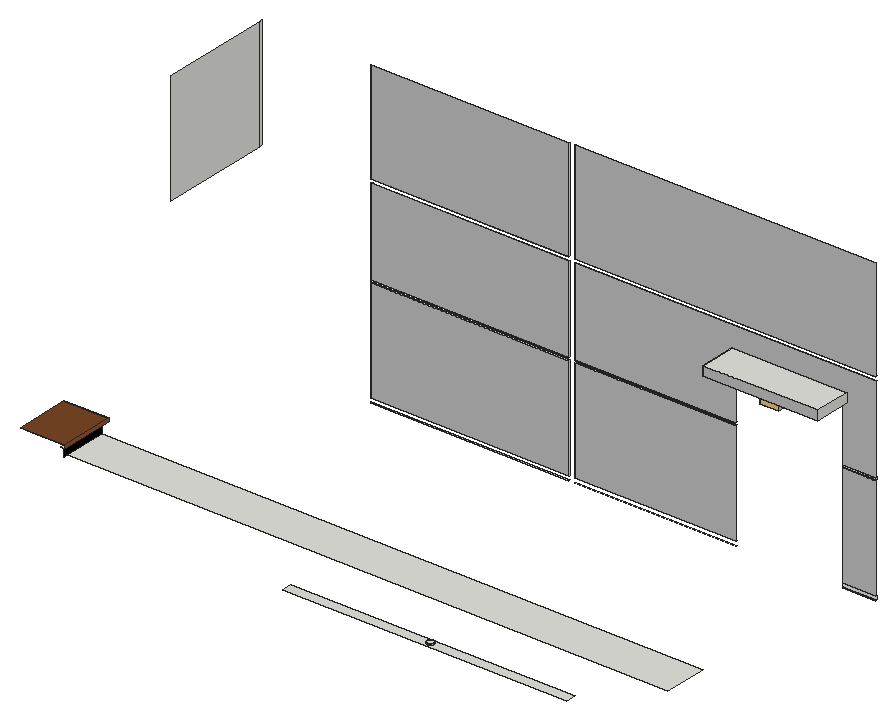
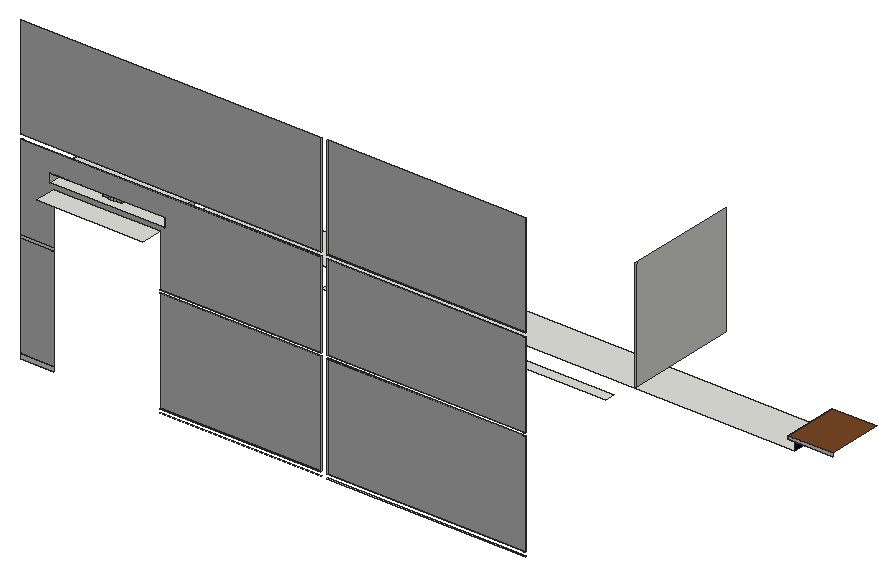
# SketchUp Ruby script. Lengths in inches.
U = 1.inch
M = Sketchup.active_model
def pt(a) = Geom::Point3d.new(a.map { |v| v * U })
def face(e, loops, mat)
  f = e.add_face(loops[0].map { |a| pt(a) })
  loops[1..].each { |l| e.add_face(l.map { |a| pt(a) }).erase! }
  f.material = f.back_material = mat if mat
  f
end
# faces: each face lists its corners as indices into pts; further lists are holes
def faces(e, pts, list, mat = nil) = list.each { |f| face(e, (f[0].is_a?(Array) ? f : [f]).map { |l| l.map { |i| pts[i] } }, mat) }
# xy, xz, yz: faces in a plane at the given z, y or x. An outline is a flat list of corners, or four numbers for a rectangle; further outlines are holes
def ring(l) = l.size == 4 ? [[l[0], l[1]], [l[2], l[1]], [l[2], l[3]], [l[0], l[3]]] : l.each_slice(2).to_a
def flat(e, list, mat, &to3) = list.each { |f| face(e, (f[0].is_a?(Array) ? f : [f]).map { |l| ring(l).map { |u, v| to3.(u, v) } }, mat) }
def xy(e, z, list, mat = nil) = flat(e, list, mat) { |x, y| [x, y, z] }
def xz(e, y, list, mat = nil) = flat(e, list, mat) { |x, z| [x, y, z] }
def yz(e, x, list, mat = nil) = flat(e, list, mat) { |y, z| [x, y, z] }
def lines(e, pts, list) = list.each { |a, b| e.add_line(pt(pts[a]), pt(pts[b])) }
# prism: a flat outline (further loops are holes) pulled along v
def prism(e, loops, v, mat = nil)
  f = face(e, loops, mat); d = Geom::Vector3d.new(v.map { |x| x * U })
  f.pushpull(f.normal.samedirection?(d) ? d.length : -d.length)
end
def box(e, o, s, mat = nil) = prism(e, [[o, [o[0] + s[0], o[1], o[2]], [o[0] + s[0], o[1] + s[1], o[2]], [o[0], o[1] + s[1], o[2]]]], [0, 0, s[2]], mat)
def at(x, y, z, deg = 0) = Geom::Transformation.translation(pt([x, y, z])) * Geom::Transformation.rotation(ORIGIN, Z_AXIS, deg.degrees)
def axes(o, x, y, z) = Geom::Transformation.new([*x, 0, *y, 0, *z, 0, *pt(o).to_a, 1])
def part(name) = M.definitions.add(name)
# library, detail: a bought-in or finely detailed component or shape, given as its bounding box
def library(name, o, s) = part(name).tap { |d| box(d.entities, o, s) }
def detail(e, o, s) = box(e.add_group.entities, o, s)
def put(e, d, t, mat = nil) = e.add_instance(d, t).tap { |i| i.material = mat if mat }
def group(e, t, mat = nil) = e.add_group.tap { |g| g.transformation = t; g.material = mat if mat }.entities
root = M.entities
M.materials.add("[0042_Sienna]1").color = [160, 82, 45]
M.materials.add("[0131_Silver]").color = [192, 192, 192]
M.materials.add("[0137_Black]").color = [0, 0, 0]
M.materials.add("[Wood Veneer 01]").color = [120, 70, 37]
c1 = library("A$C06767DEF\#1",[-8.3,1.21,0],[7.09,7.09,5.51])
xy(root,49.75,[[[765.78,333.31,873.91,337.06],[820.37,334.03,820.71,334.07,821.03,334.2,821.3,334.41,821.51,334.68,821.64,335,821.68,335.34,821.64,335.68,821.51,336,821.3,336.27,821.03,336.48,820.71,336.61,820.37,336.65,820.03,336.61,819.71,336.48,819.44,336.27,819.23,336,819.1,335.68,819.06,335.34,819.1,335,819.23,334.68,819.44,334.41,819.71,334.2,820.03,334.07]]])
xy(root,50.1875,[[820.37,334.03,820.03,334.07,819.71,334.2,819.44,334.41,819.23,334.68,819.1,335,819.06,335.34,819.1,335.68,819.23,336,819.44,336.27,819.71,336.48,820.03,336.61,820.37,336.65,820.71,336.61,821.03,336.48,821.3,336.27,821.51,336,821.64,335.68,821.68,335.34,821.64,335,821.51,334.68,821.3,334.41,821.03,334.2,820.71,334.07]])
xy(root,54.15,[[720.28,431.86,795.91,432.24],[798.1,431.86,859.31,432.24],[899.81,431.86,912.4375,432.24]])
xy(root,55.72,[[720.28,431.86,795.91,432.24],[798.1,431.86,859.31,432.24],[899.81,431.86,912.4375,432.24]])
xy(root,66.6875,[[683.8,331.81,683.875,331.81,683.875,333.31,912.4375,333.31,912.4375,349.54,683.8,349.54]])
xy(root,70.8125,[[683.8,330.31,685.3,333.31],[669.83,331.81,683.8,349.54],[683.8,333.31,685.3,351.04],[669.83,349.54,683.8,351.04]])
xy(root,72,[[668.33,330.31,685.3,351.04]],"[Wood Veneer 01]")
xy(root,95.09,[[720.28,431.86,795.91,432.24],[798.1,431.86,859.31,432.24],[899.81,431.86,912.4375,432.24]])
xy(root,96.15,[[720.28,431.86,795.91,432.24],[798.1,431.86,859.31,432.24],[899.81,431.86,912.4375,432.24]])
xy(root,115.98,[[859.31,431.86,899.81,440.22]])
xy(root,117.61,[[[857.9,418.05,901.4,431.86],[880.89,421.92,881.73,422.03,882.51,422.35,883.1875,422.87,883.7,423.54,884.03,424.33,884.14,425.17,884.03,426.01,883.7,426.79,883.1875,427.46,882.51,427.98,881.73,428.31,880.89,428.42,880.05,428.31,879.26,427.98,878.59,427.46,878.07,426.79,877.75,426.01,877.64,425.17,877.75,424.33,878.07,423.54,878.59,422.87,879.26,422.35,880.05,422.03]]])
xy(root,119.05,[[880.89,421.92,880.05,422.03,879.26,422.35,878.59,422.87,878.07,423.54,877.75,424.33,877.64,425.17,877.75,426.01,878.07,426.79,878.59,427.46,879.26,427.98,880.05,428.31,880.89,428.42,881.73,428.31,882.51,427.98,883.1875,427.46,883.7,426.79,884.03,426.01,884.14,425.17,884.03,424.33,883.7,423.54,883.1875,422.87,882.51,422.35,881.73,422.03]])
xy(root,121.23,[[857.9,418.05,901.4,431.86]])
xy(root,128.97,[[720.28,431.86,795.91,432.24],[798.1,431.86,912.4375,432.24]])
xy(root,130.53,[[720.28,431.86,795.91,432.24],[798.1,431.86,912.4375,432.24]])
xz(root,351.04,[[668.33,70.8125,685.3,72]])
xz(root,418.05,[[857.9,117.61,901.4,121.23]],"[0131_Silver]")
xz(root,431.86,[[720.28,55.72,795.91,95.09],[798.1,55.72,859.31,95.09],[899.81,55.72,912.4375,95.09],[720.28,96.15,795.91,128.97],[[798.1,96.15,859.31,96.15,859.31,115.98,899.81,115.98,899.81,96.15,912.4375,96.15,912.4375,128.97,798.1,128.97],[857.9,117.61,901.4,121.23]],
  [720.28,130.53,795.91,169.25],[798.1,130.53,912.4375,169.25]],"[0131_Silver]")
xz(root,432.24,[[899.81,54.15,912.4375,55.72],[899.81,95.09,912.4375,96.15]])
yz(root,678.11,[[389.67,126.6875,431.86,169.25],[431.86,126.6875,433.11,169.25]])
yz(root,683.8,[[331.81,66.6875,349.54,70.8125]],"[0137_Black]")
yz(root,685.3,[[330.31,70.8125,351.04,72]],"[0042_Sienna]1")
yz(root,720.28,[[431.86,55.72,432.24,95.09],[431.86,96.15,432.24,128.97],[431.86,130.53,432.24,169.25]])
yz(root,795.91,[[431.86,55.72,432.24,95.09],[431.86,96.15,432.24,128.97],[431.86,130.53,432.24,169.25]])
yz(root,798.1,[[431.86,55.72,432.24,95.09],[431.86,96.15,432.24,128.97],[431.86,130.53,432.24,169.25]])
yz(root,857.9,[[418.05,117.61,431.86,121.23]])
yz(root,901.4,[[418.05,117.61,431.86,121.23]])
p = [[820.37,334.03,49.75],[820.03,334.07,49.75],[820.03,334.07,50.1875],[820.37,334.03,50.1875],[820.71,334.07,49.75],[820.71,334.07,50.1875],
  [819.71,334.2,49.75],[819.71,334.2,50.1875],[821.03,334.2,49.75],[821.03,334.2,50.1875],[819.44,334.41,49.75],[819.44,334.41,50.1875],
  [821.3,334.41,49.75],[821.3,334.41,50.1875],[819.23,334.68,49.75],[819.23,334.68,50.1875],[821.51,334.68,49.75],[821.51,334.68,50.1875],
  [819.1,335,49.75],[819.1,335,50.1875],[821.64,335,49.75],[821.64,335,50.1875],[819.06,335.34,49.75],[819.06,335.34,50.1875],
  [821.68,335.34,49.75],[821.68,335.34,50.1875],[819.1,335.68,49.75],[819.1,335.68,50.1875],[821.64,335.68,49.75],[821.64,335.68,50.1875],
  [819.23,336,49.75],[819.23,336,50.1875],[821.51,336,49.75],[821.51,336,50.1875],[819.44,336.27,49.75],[819.44,336.27,50.1875],
  [821.3,336.27,49.75],[821.3,336.27,50.1875],[819.71,336.48,49.75],[819.71,336.48,50.1875],[821.03,336.48,49.75],[821.03,336.48,50.1875],
  [820.03,336.61,49.75],[820.03,336.61,50.1875],[820.71,336.61,49.75],[820.71,336.61,50.1875],[820.37,336.65,49.75],[820.37,336.65,50.1875],
  [880.89,421.92,117.61],[880.05,422.03,117.61],[880.05,422.03,119.05],[880.89,421.92,119.05],[881.73,422.03,117.61],[881.73,422.03,119.05],
  [879.26,422.35,117.61],[879.26,422.35,119.05],[882.51,422.35,117.61],[882.51,422.35,119.05],[878.59,422.87,117.61],[878.59,422.87,119.05],
  [883.1875,422.87,117.61],[883.1875,422.87,119.05],[878.07,423.54,117.61],[878.07,423.54,119.05],[883.7,423.54,117.61],[883.7,423.54,119.05],
  [877.75,424.33,117.61],[877.75,424.33,119.05],[884.03,424.33,117.61],[884.03,424.33,119.05],[877.64,425.17,117.61],[877.64,425.17,119.05],
  [884.14,425.17,117.61],[884.14,425.17,119.05],[877.75,426.01,117.61],[877.75,426.01,119.05],[884.03,426.01,117.61],[884.03,426.01,119.05],
  [878.07,426.79,117.61],[878.07,426.79,119.05],[883.7,426.79,117.61],[883.7,426.79,119.05],[878.59,427.46,117.61],[878.59,427.46,119.05],
  [883.1875,427.46,117.61],[883.1875,427.46,119.05],[879.26,427.98,117.61],[879.26,427.98,119.05],[882.51,427.98,117.61],[882.51,427.98,119.05],
  [880.05,428.31,117.61],[880.05,428.31,119.05],[881.73,428.31,117.61],[881.73,428.31,119.05],[880.89,428.42,117.61],[880.89,428.42,119.05]]
faces(root,p,[[0,1,2,3],[4,0,3,5],[1,6,7,2],[8,4,5,9],[6,10,11,7],[12,8,9,13],[10,14,15,11],[16,12,13,17],
  [14,18,19,15],[20,16,17,21],[18,22,23,19],[24,20,21,25],[22,26,27,23],[28,24,25,29],[26,30,31,27],[32,28,29,33],
  [30,34,35,31],[36,32,33,37],[34,38,39,35],[40,36,37,41],[38,42,43,39],[44,40,41,45],[42,46,47,43],[46,44,45,47],
  [48,49,50,51],[52,48,51,53],[49,54,55,50],[56,52,53,57],[54,58,59,55],[60,56,57,61],[58,62,63,59],[64,60,61,65],
  [62,66,67,63],[68,64,65,69],[66,70,71,67],[72,68,69,73],[70,74,75,71],[76,72,73,77],[74,78,79,75],[80,76,77,81],
  [78,82,83,79],[84,80,81,85],[82,86,87,83],[88,84,85,89],[86,90,91,87],[92,88,89,93],[90,94,95,91],[94,92,93,95]])
put(root,c1,at(885.55,419.72,113.78))
